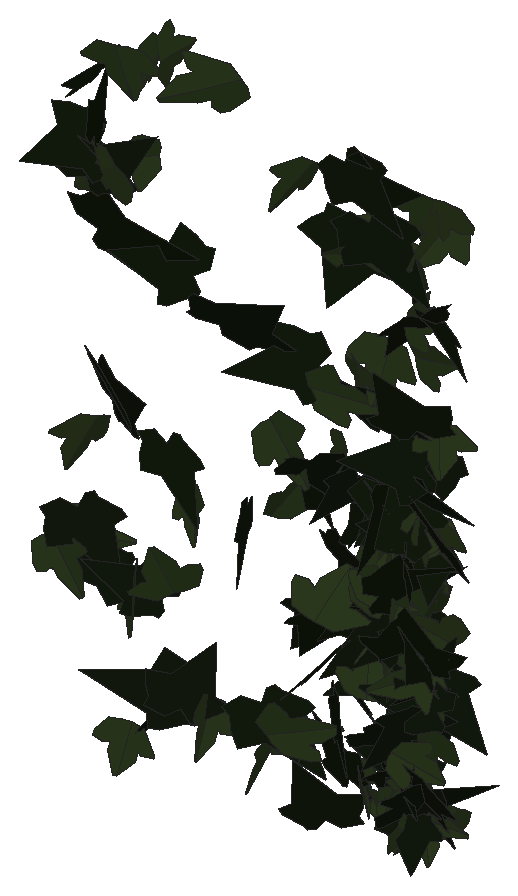
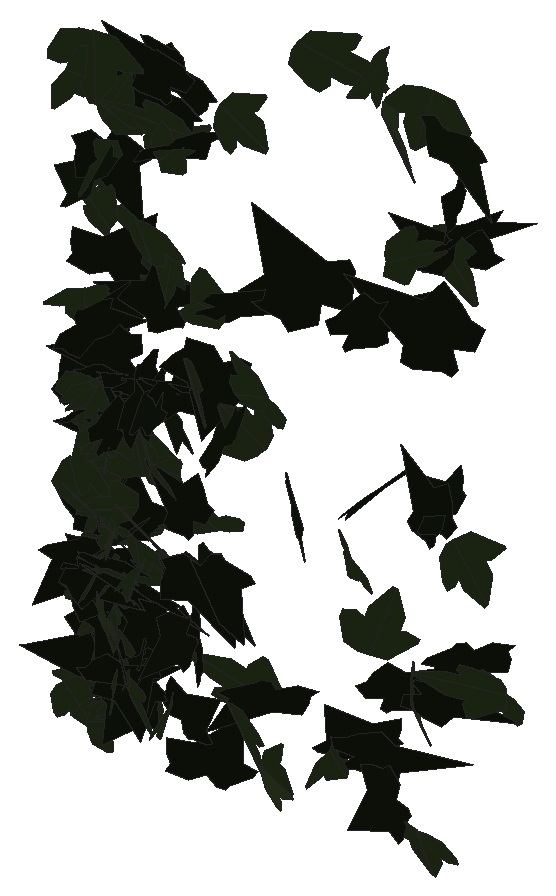
# SketchUp Ruby script. Lengths in inches.
U = 1.inch
M = Sketchup.active_model
def pt(a) = Geom::Point3d.new(a.map { |v| v * U })
def face(e, loops, mat)
  f = e.add_face(loops[0].map { |a| pt(a) })
  loops[1..].each { |l| e.add_face(l.map { |a| pt(a) }).erase! }
  f.material = f.back_material = mat if mat
  f
end
# faces: each face lists its corners as indices into pts; further lists are holes
def faces(e, pts, list, mat = nil) = list.each { |f| face(e, (f[0].is_a?(Array) ? f : [f]).map { |l| l.map { |i| pts[i] } }, mat) }
# xy, xz, yz: faces in a plane at the given z, y or x. An outline is a flat list of corners, or four numbers for a rectangle; further outlines are holes
def ring(l) = l.size == 4 ? [[l[0], l[1]], [l[2], l[1]], [l[2], l[3]], [l[0], l[3]]] : l.each_slice(2).to_a
def flat(e, list, mat, &to3) = list.each { |f| face(e, (f[0].is_a?(Array) ? f : [f]).map { |l| ring(l).map { |u, v| to3.(u, v) } }, mat) }
def xy(e, z, list, mat = nil) = flat(e, list, mat) { |x, y| [x, y, z] }
def xz(e, y, list, mat = nil) = flat(e, list, mat) { |x, z| [x, y, z] }
def yz(e, x, list, mat = nil) = flat(e, list, mat) { |y, z| [x, y, z] }
def lines(e, pts, list) = list.each { |a, b| e.add_line(pt(pts[a]), pt(pts[b])) }
# prism: a flat outline (further loops are holes) pulled along v
def prism(e, loops, v, mat = nil)
  f = face(e, loops, mat); d = Geom::Vector3d.new(v.map { |x| x * U })
  f.pushpull(f.normal.samedirection?(d) ? d.length : -d.length)
end
def box(e, o, s, mat = nil) = prism(e, [[o, [o[0] + s[0], o[1], o[2]], [o[0] + s[0], o[1] + s[1], o[2]], [o[0], o[1] + s[1], o[2]]]], [0, 0, s[2]], mat)
def at(x, y, z, deg = 0) = Geom::Transformation.translation(pt([x, y, z])) * Geom::Transformation.rotation(ORIGIN, Z_AXIS, deg.degrees)
def axes(o, x, y, z) = Geom::Transformation.new([*x, 0, *y, 0, *z, 0, *pt(o).to_a, 1])
def part(name) = M.definitions.add(name)
# library, detail: a bought-in or finely detailed component or shape, given as its bounding box
def library(name, o, s) = part(name).tap { |d| box(d.entities, o, s) }
def detail(e, o, s) = box(e.add_group.entities, o, s)
def put(e, d, t, mat = nil) = e.add_instance(d, t).tap { |i| i.material = mat if mat }
def group(e, t, mat = nil) = e.add_group.tap { |g| g.transformation = t; g.material = mat if mat }.entities
root = M.entities
M.materials.add("1026 AP 7946 SUNNY SIDE UP").color = [254, 231, 186]
M.materials.add("efeu1").color = [18, 25, 13]
M.materials.add("efeu2").color = [43, 57, 29]
c1 = part("ivyleaf_9")
p = [[1.54,2.16,1.25],[1.36,2.04,1.19],[-0.21,0.99,0.68],[-0.71,1.11,0.82],[-0.85,0.86,0.67],[-0.8,0.17,0.21],
  [-0.9,-0.01,0.1],[-0.67,-0.16,-0.02],[-0.08,-0.08,-0.05],[-0.03,-0.6,-0.4],[0.65,-0.88,-0.66],[0.83,-0.6,-0.49],
  [1.29,-0.42,-0.43],[1.8125,-0.07,-0.26],[1.21,0.44,0.15]]
faces(c1.entities,p,[[0,1,2,3,4,5,6,7,8,9,10,11,12,13,14]],"efeu1")
c2 = part("ivyleaf_10")
p = [[0,0.5,-0.03],[-0.0625,2.02,-0.43],[-0.19,2.01,-0.46],[-0.54,1.05,-0.29],[-0.52,0.625,-0.18],[-0.83,0.76,-0.28],
  [-1.16,0.64,-0.33],[-1.15,0.33,-0.24],[-0.77,-0.39,0.02],[-0.3,-0.51,0.16],[0.04,-0.48,0.23],[-0.02,2.01,-0.4375],
  [-0.06,2.01,-0.43],[0.04,-0.49,0.23],[0.67,-0.49,0.14],[1.38,0.36,-0.2],[1.375,0.51,-0.24],[0.81,0.65,-0.19],
  [0.62,0.59,-0.15],[0.6,1.09,-0.28],[0.5,1.23,-0.31]]
faces(c2.entities,p,[[0,1,2,3,4,5,6,7,8,9,10],[11,12,0,13,14,15,16,17,18,19,20]],"efeu2")
put(root,c1,axes([136.73,210.17,270.59],[-0.26614,0.28728,-0.15175],[0.0914,-0.13835,-0.34379],[-0.50054,-0.17801,0.01791]),"1026 AP 7946 SUNNY SIDE UP")
put(root,c1,axes([134.75,210.21,275.29],[0.64313,0.07781,-0.06027],[0.07787,0.05342,0.42695],[0.13227,-0.40977,0.04169]),"1026 AP 7946 SUNNY SIDE UP")
put(root,c1,axes([138.13,210.27,268.39],[-0.27927,-0.11413,-0.14956],[0.23344,0.03006,-0.21224],[0.17132,-0.227,0.0454]),"1026 AP 7946 SUNNY SIDE UP")
put(root,c1,axes([137.875,209.9,272.13],[0.11299,0.0966,0.37841],[0.47621,0.2101,-0.11691],[-0.35901,0.3091,-0.03598]),"1026 AP 7946 SUNNY SIDE UP")
put(root,c1,axes([138.1,210.46,271.06],[-0.02512,-0.18644,0.31261],[-0.05138,-0.30277,-0.19451],[0.55907,-0.03621,-0.00383]),"1026 AP 7946 SUNNY SIDE UP")
put(root,c2,axes([134.65,210.36,279.11],[-0.23805,-0.09443,0.34964],[-0.35505,-0.25829,-0.17903],[0.42625,-0.26788,0.04614]),"1026 AP 7946 SUNNY SIDE UP")
put(root,c2,axes([138.25,210.43,270.72],[0.13107,0.05274,-0.3635],[-0.35701,-0.27206,-0.09866],[-0.43333,0.2401,-0.02867]),"1026 AP 7946 SUNNY SIDE UP")
put(root,c1,axes([132.18,210.5,277.25],[-0.2853,-0.16132,0.29209],[-0.28268,-0.22252,-0.24944],[0.42951,-0.2536,0.02985]),"1026 AP 7946 SUNNY SIDE UP")
put(root,c1,axes([133.65,210.33,272.86],[0.10695,-0.35729,-0.04746],[-0.02162,0.04221,-0.3744],[0.56564,0.06917,-0.00534]),"1026 AP 7946 SUNNY SIDE UP")
put(root,c2,axes([135.89,210.13,272.75],[-0.05032,-0.28781,0.17373],[0.02448,0.16958,0.29931],[-0.52525,0.03548,-0.00269]),"1026 AP 7946 SUNNY SIDE UP")
put(root,c2,axes([133.69,210.36,270.61],[-0.30833,-0.26039,-0.16424],[-0.18219,-0.10995,0.33427],[-0.44287,0.22652,-0.02316]),"1026 AP 7946 SUNNY SIDE UP")
put(root,c2,axes([138.125,210.37,268.875],[-0.10338,-0.1906,0.18428],[-0.07209,-0.17431,-0.20847],[0.40582,-0.07952,0.00991]),"1026 AP 7946 SUNNY SIDE UP")
put(root,c1,axes([138.22,210.375,269.99],[-0.01066,0.16452,-0.33169],[-0.00555,-0.32297,-0.17134],[-0.56981,0.00007,0.00788]),"1026 AP 7946 SUNNY SIDE UP")
put(root,c1,axes([136.56,210.45,269.68],[-0.03088,-0.02035,-0.38486],[0.54423,-0.14274,-0.01158],[-0.22291,-0.34568,0.02506]),"1026 AP 7946 SUNNY SIDE UP")
put(root,c2,axes([138.13,210.07,269.46],[0.12399,0.16893,0.25185],[0.1136,0.23342,-0.18956],[-0.45195,0.10502,0.02144]),"1026 AP 7946 SUNNY SIDE UP")
put(root,c1,axes([134.97,210.46,272.2],[-0.19885,0.023,-0.35438],[0.47826,-0.16535,-0.12751],[-0.25566,-0.32722,0.03711]),"1026 AP 7946 SUNNY SIDE UP")
put(root,c1,axes([133.89,210.39,268.8],[-0.27735,0.03023,0.33699],[-0.51531,-0.03891,-0.17867],[0.03157,-0.36945,0.04419]),"1026 AP 7946 SUNNY SIDE UP")
put(root,c2,axes([135.83,210.19,269.01],[-0.25935,-0.06483,0.30417],[0.39299,0.1607,0.1809],[-0.26838,0.29795,-0.02905]),"1026 AP 7946 SUNNY SIDE UP")
put(root,c2,axes([137.25,210.25,271.875],[-0.00984,0.02412,0.31447],[0.46837,0.07065,0.00095],[-0.11066,0.29689,-0.02393]),"1026 AP 7946 SUNNY SIDE UP")
put(root,c1,axes([138.06,210.5625,273.98],[-0.18142,-0.07753,0.38218],[-0.43482,-0.24863,-0.14341],[0.40851,-0.29908,0.01708]),"1026 AP 7946 SUNNY SIDE UP")
put(root,c2,axes([131.58,210.34,270.52],[0.37526,-0.01701,0.23964],[0.36328,-0.02943,-0.24647],[0.05143,0.33203,-0.00761]),"1026 AP 7946 SUNNY SIDE UP")
put(root,c1,axes([136.43,210.13,273.68],[0.30385,0.27277,-0.0482],[-0.02167,-0.04939,-0.34421],[-0.43505,0.19297,-0.01652]),"1026 AP 7946 SUNNY SIDE UP")
put(root,c2,axes([132.83,210.28,278.96],[-0.52336,-0.04407,-0.04314],[0.07175,-0.0292,-0.34421],[0.06275,-0.33416,0.03377]),"1026 AP 7946 SUNNY SIDE UP")
put(root,c2,axes([132.86,210.37,267.92],[0.47079,-0.06296,0.02228],[0.02472,-0.03166,-0.31409],[0.10191,0.29854,-0.02676]),"1026 AP 7946 SUNNY SIDE UP")
put(root,c1,axes([137.97,210.37,270.9],[0.51186,0.03665,0.18094],[-0.28073,0.03454,0.33405],[0.02463,-0.36817,0.04716]),"1026 AP 7946 SUNNY SIDE UP")
put(root,c2,axes([137.99,210.44,272.24],[0.15379,0.23935,-0.21078],[-0.09836,-0.19665,-0.26719],[-0.48667,0.11538,-0.01261]),"1026 AP 7946 SUNNY SIDE UP")
put(root,c1,axes([138.04,210.22,269.12],[0.63379,-0.06727,-0.16095],[-0.24931,-0.00577,-0.41991],[0.09533,0.43212,-0.02808]),"1026 AP 7946 SUNNY SIDE UP")
put(root,c2,axes([135.49,210.44,273.6875],[0.33715,-0.01288,0.33394],[0.49072,-0.09821,-0.21722],[0.13969,0.3761,-0.04293]),"1026 AP 7946 SUNNY SIDE UP")
put(root,c1,axes([138.08,210.4,274.6875],[0.2781,0.01571,0.27956],[-0.42679,0.02574,0.18092],[-0.0205,-0.32282,0.02613]),"1026 AP 7946 SUNNY SIDE UP")
put(root,c1,axes([137.61,210.56,268.89],[0.09588,-0.22587,0.23585],[0.08395,-0.224,-0.24228],[0.50014,0.0809,-0.00455]),"1026 AP 7946 SUNNY SIDE UP")
put(root,c2,axes([137.99,210.2,268.24],[-0.06269,-0.1766,-0.22164],[0.12216,0.20059,-0.18415],[0.41901,-0.08491,0.02053]),"1026 AP 7946 SUNNY SIDE UP")
put(root,c1,axes([138.45,210.36,270.23],[-0.25328,0.0694,0.2497],[-0.37256,0.05528,-0.17849],[-0.13376,-0.28539,0.02432]),"1026 AP 7946 SUNNY SIDE UP")
put(root,c1,axes([134.01,210.2,268.83],[-0.29691,-0.04659,0.28487],[0.39529,0.1203,0.19824],[-0.1963,0.31272,-0.03168]),"1026 AP 7946 SUNNY SIDE UP")
put(root,c1,axes([136.92,210.49,273.4],[-0.04346,0.10021,-0.27693],[0.0868,-0.26374,-0.10845],[-0.44353,-0.06143,0.00592]),"1026 AP 7946 SUNNY SIDE UP")
put(root,c2,axes([134.3,210.5,268.74],[0.06042,0.28703,-0.22609],[-0.06918,-0.21699,-0.29935],[-0.56548,0.05721,0.01247]),"1026 AP 7946 SUNNY SIDE UP")
put(root,c1,axes([138.32,210.34,268.61],[0.12464,-0.0563,0.25825],[-0.29095,0.16998,0.10047],[-0.28099,-0.20098,0.01052]),"1026 AP 7946 SUNNY SIDE UP")
put(root,c1,axes([138.06,210.24,272.6],[0.17787,-0.10591,-0.28495],[-0.35878,0.15661,-0.15734],[0.29554,0.25386,-0.01952]),"1026 AP 7946 SUNNY SIDE UP")
put(root,c2,axes([137.28,210.29,270.23],[0.35223,0.16172,-0.04466],[0.03139,0.04762,0.28359],[0.26177,-0.22332,0.02608]),"1026 AP 7946 SUNNY SIDE UP")
put(root,c1,axes([138,210.09,268.62],[0.11303,0.31226,-0.27155],[0.04457,0.26498,0.33068],[0.6428,-0.07328,0.02482]),"1026 AP 7946 SUNNY SIDE UP")
put(root,c2,axes([138.37,210.35,269.82],[-0.48773,0.03857,0.12281],[-0.19078,-0.0154,-0.32078],[-0.04783,-0.33187,0.02718]),"1026 AP 7946 SUNNY SIDE UP")
put(root,c1,axes([137.25,210.45,277.66],[-0.13024,-0.14572,-0.36707],[0.52719,0.15015,-0.14301],[0.29498,-0.33269,0.09352]),"1026 AP 7946 SUNNY SIDE UP")
put(root,c1,axes([132.47,210.26,278.6],[-0.17953,0.34768,0.01294],[-0.02468,0.00598,-0.37672],[-0.54639,-0.11451,0.01276]),"1026 AP 7946 SUNNY SIDE UP")
put(root,c1,axes([136.08,210.62,274.91],[-0.38108,-0.0838,0.26753],[-0.34164,-0.1519,-0.2598],[0.26076,-0.32148,0.05059]),"1026 AP 7946 SUNNY SIDE UP")
put(root,c2,axes([136.52,210.22,271.27],[0.46457,0.1013,-0.15908],[0.14876,0.1683,0.3001],[0.25027,-0.28808,0.11692]),"1026 AP 7946 SUNNY SIDE UP")
put(root,c1,axes([135.37,210.35,269.24],[0.03333,-0.25357,-0.28363],[0.11211,0.27202,-0.25217],[0.57607,-0.03827,0.06549]),"1026 AP 7946 SUNNY SIDE UP")
put(root,c2,axes([132.58,210.35,276.98],[-0.41771,0.07158,0.26406],[-0.40832,0.0069,-0.27964],[-0.08871,-0.3688,0.04378]),"1026 AP 7946 SUNNY SIDE UP")
put(root,c1,axes([138.15,210.37,276.5],[-0.03699,0.31016,-0.14915],[0.0141,-0.14628,-0.32129],[-0.5392,-0.0251,0.00183]),"1026 AP 7946 SUNNY SIDE UP")
put(root,c1,axes([137.39,210.72,273.2],[-0.04348,-0.01088,-0.46251],[0.46618,-0.33821,-0.01234],[-0.53026,-0.29645,0.02707]),"1026 AP 7946 SUNNY SIDE UP")
put(root,c2,axes([137.78,210.33,268.42],[0.0358,0.01827,0.38531],[0.53357,0.1572,-0.02828],[-0.24861,0.34003,-0.00521]),"1026 AP 7946 SUNNY SIDE UP")
put(root,c1,axes([137.34,210.23,269.54],[0.28308,0.18338,0.10229],[0.13226,0.05467,-0.26359],[-0.29919,0.19767,-0.01975]),"1026 AP 7946 SUNNY SIDE UP")
put(root,c2,axes([137.6,210.3125,271.8],[0.4458,0.18264,-0.07887],[0.07595,0.06772,0.34646],[0.30264,-0.28603,0.02922]),"1026 AP 7946 SUNNY SIDE UP")
put(root,c2,axes([137.34,210.44,268.4],[-0.28245,0.15267,-0.1004],[0.09622,-0.07932,-0.24252],[-0.26884,-0.18879,0.01868]),"1026 AP 7946 SUNNY SIDE UP")
put(root,c2,axes([136.43,210.39,274.68],[-0.08928,0.00465,0.35232],[0.51863,0.09238,0.05566],[-0.14215,0.33411,-0.01819]),"1026 AP 7946 SUNNY SIDE UP")
put(root,c1,axes([136.38,210.48,267.73],[0.26833,0.08542,0.26178],[-0.4152,0.0048,0.1814],[0.06847,-0.30565,0.07408]),"1026 AP 7946 SUNNY SIDE UP")
put(root,c2,axes([138.46,210.6,271.29],[-0.21494,-0.15184,-0.27938],[-0.34525,-0.16119,0.2067],[-0.34422,0.25648,-0.03287]),"1026 AP 7946 SUNNY SIDE UP")
put(root,c2,axes([132.05,210.55,272.5625],[-0.13776,-0.34154,0.11707],[-0.02345,-0.11541,-0.36365],[0.56647,-0.08784,0.01342]),"1026 AP 7946 SUNNY SIDE UP")
put(root,c2,axes([136.91,210.68,276.97],[-0.07115,-0.06947,-0.31803],[-0.22034,-0.27477,0.08336],[-0.44544,0.14701,0.00957]),"1026 AP 7946 SUNNY SIDE UP")
put(root,c1,axes([132.23,210.33,276.79],[-0.15861,0.02976,0.32855],[0.50332,0.01482,0.10301],[-0.00821,0.334,-0.03187]),"1026 AP 7946 SUNNY SIDE UP")
put(root,c2,axes([137.39,210.57,275.6],[0.56896,-0.11957,0.04142],[0.04608,-0.04123,-0.39163],[0.19328,0.3618,-0.02857]),"1026 AP 7946 SUNNY SIDE UP")
put(root,c1,axes([137.65,210.64,273.2],[-0.40454,-0.12657,0.01914],[-0.00818,-0.03295,-0.29424],[0.20115,-0.25588,0.02654]),"1026 AP 7946 SUNNY SIDE UP")
put(root,c1,axes([138.07,210.51,273.02],[-0.44402,-0.18993,-0.17658],[-0.25408,-0.06345,0.34851],[-0.31041,0.32361,-0.03268]),"1026 AP 7946 SUNNY SIDE UP")
put(root,c1,axes([137.58,210.4375,269.24],[0.29218,-0.12814,-0.15735],[-0.2256,0.05762,-0.23037],[0.21642,0.23306,-0.0277]),"1026 AP 7946 SUNNY SIDE UP")
put(root,c2,axes([138.23,210.63,271.92],[-0.07504,-0.35159,0.14809],[-0.00667,-0.14639,-0.36608],[0.59842,-0.04572,0.01449]),"1026 AP 7946 SUNNY SIDE UP")
put(root,c1,axes([137.84,210.36,269.44],[0.29876,0.18475,0.00136],[0.02017,-0.0128,-0.27245],[-0.28981,0.18957,-0.01755]),"1026 AP 7946 SUNNY SIDE UP")
put(root,c1,axes([136.75,210.76,277.17],[-0.28079,-0.33585,0.08636],[-0.02977,-0.08685,-0.39162],[0.54422,-0.17803,0.02314]),"1026 AP 7946 SUNNY SIDE UP")
put(root,c1,axes([135.87,210.77,272.97],[0.29081,-0.17782,-0.2867],[0.35119,-0.16606,0.26219],[-0.38073,-0.289,0.02286]),"1026 AP 7946 SUNNY SIDE UP")
put(root,c2,axes([138.18,210.5,268.17],[0.11528,0.23643,-0.02662],[-0.00166,-0.02812,-0.25506],[-0.3742,0.07296,-0.00707]),"1026 AP 7946 SUNNY SIDE UP")
put(root,c1,axes([137.75,210.74,270.8],[-0.12014,-0.21094,0.19055],[-0.0125,-0.19121,-0.22768],[0.4422,-0.06271,0.04533]),"1026 AP 7946 SUNNY SIDE UP")
put(root,c2,axes([138.3125,210.45,270.25],[0.14915,-0.06816,-0.26612],[-0.36169,0.11778,-0.11852],[0.21251,0.2483,-0.01494]),"1026 AP 7946 SUNNY SIDE UP")
put(root,c2,axes([137.11,210.69,272.19],[0.36911,-0.14025,0.27182],[0.30546,-0.18463,-0.2794],[0.35847,0.30175,-0.04181]),"1026 AP 7946 SUNNY SIDE UP")
put(root,c1,axes([138.4,210.6,272.73],[0.29423,-0.29874,0.18965],[-0.12962,0.16734,0.36372],[-0.53777,-0.20378,0.0161]),"1026 AP 7946 SUNNY SIDE UP")
put(root,c2,axes([137.07,210.47,275.1875],[-0.41398,0.17699,0.04124],[-0.07851,-0.00466,-0.32523],[-0.27395,-0.26611,0.03087]),"1026 AP 7946 SUNNY SIDE UP")
put(root,c1,axes([138.1,210.32,269.375],[-0.07557,0.00756,-0.34682],[-0.47051,0.15511,0.04849],[0.243,0.30268,-0.01396]),"1026 AP 7946 SUNNY SIDE UP")
put(root,c2,axes([137.91,210.7,269.83],[0.03658,-0.20463,0.20217],[0.10227,-0.18899,-0.21082],[0.43523,0.06161,0.03255]),"1026 AP 7946 SUNNY SIDE UP")
put(root,c2,axes([138,210.48,277.14],[-0.42318,0.17665,-0.11522],[-0.12491,0.084,0.33112],[0.30502,0.27948,-0.02426]),"1026 AP 7946 SUNNY SIDE UP")
put(root,c1,axes([138.15,210.6875,272.67],[-0.12286,-0.27832,0.0111],[0.00789,-0.01424,-0.29775],[0.43798,-0.07781,0.00848]),"1026 AP 7946 SUNNY SIDE UP")
put(root,c2,axes([132.65,210.76,270.16],[0.23681,-0.17536,0.32947],[0.3335,-0.24071,-0.23953],[0.46827,0.26012,0.00397]),"1026 AP 7946 SUNNY SIDE UP")
put(root,c1,axes([137.17,210.33,272.86],[-0.23097,0.0674,-0.26752],[-0.33571,0.15062,0.16533],[0.2564,0.25792,-0.02451]),"1026 AP 7946 SUNNY SIDE UP")
put(root,c1,axes([136.9,210.5625,274.6],[0.29094,-0.06199,0.22944],[0.3002,-0.12068,-0.1984],[0.20594,0.2635,-0.03494]),"1026 AP 7946 SUNNY SIDE UP")
put(root,c2,axes([137.95,210.79,268.0625],[0.01537,-0.09049,0.32955],[0.09327,-0.31494,-0.09534],[0.51514,0.05972,0.00743]),"1026 AP 7946 SUNNY SIDE UP")
put(root,c2,axes([135.78,210.72,277.93],[-0.05215,-0.27539,0.21292],[-0.02696,-0.20763,-0.2869],[0.54222,-0.03681,0.00621]),"1026 AP 7946 SUNNY SIDE UP")
put(root,c2,axes([133.76,210.68,271.9],[0.3071,-0.12001,0.21594],[0.26128,-0.13007,-0.23622],[0.2769,0.25583,-0.0166]),"1026 AP 7946 SUNNY SIDE UP")
put(root,c1,axes([138.16,210.45,270.32],[0.14353,0.25165,-0.06108],[-0.02223,-0.05944,-0.27603],[-0.40644,0.09212,-0.00647]),"1026 AP 7946 SUNNY SIDE UP")
put(root,c1,axes([132.16,210.78,273.25],[0.11308,-0.2263,0.26656],[0.11042,-0.25044,-0.246],[0.53066,0.10034,-0.00561]),"1026 AP 7946 SUNNY SIDE UP")
put(root,c1,axes([131.88,210.53,271.125],[-0.01622,-0.27492,-0.25137],[0.01182,0.24233,-0.282],[0.57624,-0.01271,-0.00129]),"1026 AP 7946 SUNNY SIDE UP")
put(root,c2,axes([133.62,210.29,279.22],[0.0346,-0.05695,-0.36877],[0.10546,0.35274,-0.05155],[0.55959,-0.06296,0.03251]),"1026 AP 7946 SUNNY SIDE UP")
put(root,c1,axes([133.16,210.71,270.11],[-0.05961,0.03673,0.34222],[-0.49032,-0.12359,-0.02332],[0.18815,-0.31044,0.04764]),"1026 AP 7946 SUNNY SIDE UP")
put(root,c1,axes([132.3,210.36,277.5],[-0.04261,-0.07348,0.33653],[0.17172,0.30831,0.08248],[-0.49837,0.11252,-0.00035]),"1026 AP 7946 SUNNY SIDE UP")
put(root,c1,axes([132.55,210.69,270.32],[-0.12236,-0.10405,-0.28652],[-0.26869,-0.2187,0.13255],[-0.38081,0.18774,-0.00146]),"1026 AP 7946 SUNNY SIDE UP")
put(root,c1,axes([132.33,210.76,272.98],[-0.01399,-0.02126,0.38076],[0.19042,-0.34966,-0.01975],[0.55029,0.12045,0.01652]),"1026 AP 7946 SUNNY SIDE UP")
put(root,c2,axes([135.11,210.76,268.28],[0.15126,-0.23356,0.22129],[0.10025,-0.20707,-0.26096],[0.49022,0.11441,-0.01491]),"1026 AP 7946 SUNNY SIDE UP")
put(root,c1,axes([137.45,210.66,271.16],[-0.60423,0.14588,-0.1043],[0.12757,-0.07266,-0.42205],[-0.24921,-0.3909,0.03684]),"1026 AP 7946 SUNNY SIDE UP")
put(root,c1,axes([133.67,210.81,275.46],[-0.10197,-0.00874,0.39409],[-0.48887,-0.22504,-0.06091],[0.35084,-0.31612,0.02967]),"1026 AP 7946 SUNNY SIDE UP")
put(root,c1,axes([132.18,210.68,275.72],[0.2045,-0.0656,0.4257],[0.50475,-0.2625,-0.14841],[0.42285,0.34506,-0.02872]),"1026 AP 7946 SUNNY SIDE UP")
put(root,c1,axes([137.67,210.6,273.55],[0.33403,-0.08508,0.1851],[0.25562,-0.07824,-0.236],[0.18112,0.26733,-0.0083]),"1026 AP 7946 SUNNY SIDE UP")
put(root,c2,axes([137.97,210.68,275.64],[-0.22788,0.07635,0.30345],[0.45192,-0.07136,0.16456],[0.15514,0.32003,-0.03363]),"1026 AP 7946 SUNNY SIDE UP")
put(root,c1,axes([137.92,210.73,270.24],[-0.43063,-0.05853,-0.06874],[0.1144,-0.02591,-0.28578],[0.07927,-0.2806,0.039]),"1026 AP 7946 SUNNY SIDE UP")
put(root,c2,axes([137.89,210.57,270.1],[-0.19892,-0.10465,-0.21233],[0.33933,0.02895,-0.15187],[0.12789,-0.23958,0.07271]),"1026 AP 7946 SUNNY SIDE UP")
put(root,c2,axes([138.13,210.7,273.02],[0.27167,0.19318,-0.13302],[-0.10541,-0.11403,-0.26658],[-0.35082,0.18386,-0.0229]),"1026 AP 7946 SUNNY SIDE UP")
put(root,c1,axes([137.4375,210.54,269.12],[0.23388,-0.02503,-0.22362],[-0.34013,0.01899,-0.15494],[0.04694,0.26233,-0.00856]),"1026 AP 7946 SUNNY SIDE UP")
put(root,c1,axes([137.93,210.75,270.49],[-0.35508,-0.12648,-0.05556],[0.09955,-0.00512,-0.26427],[0.19143,-0.23195,0.03437]),"1026 AP 7946 SUNNY SIDE UP")
put(root,c1,axes([136.62,210.7,278.3],[-0.06251,-0.09717,-0.34855],[0.52079,0.10344,-0.07021],[0.18501,-0.324,0.07986]),"1026 AP 7946 SUNNY SIDE UP")
put(root,c2,axes([136.94,210.61,277.28],[0.06683,-0.03585,-0.33407],[0.51219,-0.00984,0.04507],[-0.02276,-0.32671,0.03337]),"1026 AP 7946 SUNNY SIDE UP")
put(root,c2,axes([136.59,210.55,273.7],[0.17826,-0.23479,-0.19294],[-0.1228,0.16878,-0.2676],[0.45466,0.13764,0.00337]),"1026 AP 7946 SUNNY SIDE UP")
put(root,c2,axes([137.48,210.49,268.34],[0.09731,0.07064,0.24985],[0.21347,0.20077,-0.09492],[-0.33423,0.1488,0.01211]),"1026 AP 7946 SUNNY SIDE UP")
put(root,c1,axes([136.87,210.72,278.03],[0.0513,-0.00636,0.32549],[0.34867,-0.22589,-0.02959],[0.35411,0.22334,-0.01802]),"1026 AP 7946 SUNNY SIDE UP")
put(root,c1,axes([137.24,210.7,270.26],[-0.40373,0.04838,0.03375],[-0.05535,-0.01181,-0.2686],[-0.07303,-0.25854,0.01702]),"1026 AP 7946 SUNNY SIDE UP")
put(root,c2,axes([138.1,210.68,272.96],[0.10453,0.27439,-0.07754],[-0.01393,-0.07686,-0.29114],[-0.44782,0.06644,-0.00904]),"1026 AP 7946 SUNNY SIDE UP")
put(root,c2,axes([137.32,210.73,270.92],[0.39962,-0.07196,0.08405],[0.11071,-0.0506,-0.27086],[0.13103,0.26221,-0.0275]),"1026 AP 7946 SUNNY SIDE UP")
put(root,c2,axes([137.91,210.58,269.24],[0.29501,-0.12811,-0.17486],[-0.15163,0.14944,-0.22611],[0.297,0.20355,0.05825]),"1026 AP 7946 SUNNY SIDE UP")
put(root,c2,axes([136.9,210.69,268.57],[-0.08496,0.28251,-0.09695],[0.0206,-0.09493,-0.29683],[-0.46857,-0.0554,0.00453]),"1026 AP 7946 SUNNY SIDE UP")
put(root,c2,axes([137.9375,210.72,269.86],[0.07932,-0.25559,0.02896],[0.0059,-0.02939,-0.26855],[0.40453,0.05055,-0.00176]),"1026 AP 7946 SUNNY SIDE UP")
put(root,c2,axes([137.71,210.6,268.82],[0.02969,-0.25103,-0.12555],[0.0899,0.12165,-0.25124],[0.42848,-0.00813,0.06142]),"1026 AP 7946 SUNNY SIDE UP")
put(root,c1,axes([136.69,210.6,268.48],[0.09698,-0.06919,0.276],[-0.21527,0.23136,0.09524],[-0.37878,-0.1492,0.01653]),"1026 AP 7946 SUNNY SIDE UP")
put(root,c2,axes([137.93,210.67,272.46],[-0.38206,-0.0209,-0.13597],[0.2099,-0.03275,-0.24823],[0.00405,-0.27451,0.03833]),"1026 AP 7946 SUNNY SIDE UP")
put(root,c1,axes([138.16,210.95,274.04],[0.00275,-0.12571,-0.32902],[0.11359,-0.31136,0.12513],[-0.52653,-0.06783,0.02527]),"1026 AP 7946 SUNNY SIDE UP")
put(root,c2,axes([131.59,210.6,270.68],[0.03832,-0.05803,-0.35269],[0.5398,0.05339,0.01618],[0.07852,-0.33871,0.06089]),"1026 AP 7946 SUNNY SIDE UP")
put(root,c1,axes([133.3125,210.39,268.34],[0.12751,0.18232,0.29102],[0.18399,0.25598,-0.20406],[-0.49415,0.14236,-0.00089]),"1026 AP 7946 SUNNY SIDE UP")
put(root,c2,axes([137.78,210.49,271.24],[-0.02813,-0.01088,0.28642],[0.09509,0.27185,0.01656],[-0.42715,0.06124,-0.01518]),"1026 AP 7946 SUNNY SIDE UP")
put(root,c2,axes([137.89,210.68,270.91],[-0.22698,0.21919,-0.05018],[0.02875,-0.04772,-0.27043],[-0.35232,-0.14511,0.01026]),"1026 AP 7946 SUNNY SIDE UP")
put(root,c1,axes([138.25,210.79,270.25],[-0.16494,0.11927,-0.21148],[0.00944,-0.22368,-0.1379],[-0.37411,-0.05823,0.08976]),"1026 AP 7946 SUNNY SIDE UP")
put(root,c1,axes([138.09,210.61,270.48],[-0.06414,-0.20871,-0.33973],[0.1244,0.31905,-0.21702],[0.59932,-0.08856,0.00869]),"1026 AP 7946 SUNNY SIDE UP")
put(root,c2,axes([138.29,210.91,277.8],[0.13271,0.22612,-0.32987],[-0.22091,-0.28974,-0.24963],[-0.57719,0.16288,0.0197]),"1026 AP 7946 SUNNY SIDE UP")
put(root,c1,axes([136.35,210.86,271.74],[0.08373,-0.0757,0.3132],[0.23371,-0.26586,-0.09644],[0.43441,0.15762,-0.00848]),"1026 AP 7946 SUNNY SIDE UP")
put(root,c1,axes([138.28,210.79,271.29],[-0.40064,0.05505,-0.1023],[0.1405,-0.05452,-0.26681],[-0.11085,-0.26809,0.03155]),"1026 AP 7946 SUNNY SIDE UP")
put(root,c2,axes([138.43,210.8,268.36],[-0.18061,-0.21018,0.12151],[-0.06895,-0.1116,-0.24702],[0.37359,-0.12221,0.01315]),"1026 AP 7946 SUNNY SIDE UP")
put(root,c2,axes([138.04,210.45,276.33],[-0.01913,0.08193,0.33741],[-0.12041,0.31804,-0.08315],[-0.5163,-0.07721,0.00689]),"1026 AP 7946 SUNNY SIDE UP")
put(root,c1,axes([137.69,210.99,272.55],[-0.08553,-0.03052,0.39146],[-0.38051,-0.29404,-0.06171],[0.4635,-0.24702,0.02158]),"1026 AP 7946 SUNNY SIDE UP")
put(root,c2,axes([138.15,210.71,278.15],[-0.57095,-0.07429,0.04535],[-0.06093,-0.03186,-0.38125],[0.12172,-0.36443,0.02185]),"1026 AP 7946 SUNNY SIDE UP")
put(root,c1,axes([136.3,210.7,270.91],[0.09091,0.27104,-0.19786],[-0.04841,-0.1913,-0.2865],[-0.52149,0.06501,-0.00789]),"1026 AP 7946 SUNNY SIDE UP")
put(root,c1,axes([137.54,210.63,268.76],[0.14602,0.21927,-0.08849],[-0.0828,-0.07203,-0.24494],[-0.36165,0.10502,0.02035]),"1026 AP 7946 SUNNY SIDE UP")
put(root,c1,axes([136.27,210.73,270.9375],[0.20083,0.15156,-0.2685],[-0.24102,-0.21218,-0.20507],[-0.40959,0.19917,-0.01098]),"1026 AP 7946 SUNNY SIDE UP")
put(root,c1,axes([137.97,210.91,276.28],[0.16927,-0.29437,0.16188],[0.10009,-0.14575,-0.32363],[0.51632,0.12476,0.00967]),"1026 AP 7946 SUNNY SIDE UP")
put(root,c1,axes([137.8,210.83,268.75],[-0.07265,0.02946,0.29003],[-0.44056,-0.04419,-0.04289],[0.06152,-0.28169,0.03535]),"1026 AP 7946 SUNNY SIDE UP")
put(root,c2,axes([135.67,210.72,268.91],[0.35976,-0.27291,-0.144],[-0.15613,0.09702,-0.36607],[0.45498,0.24908,-0.01176]),"1026 AP 7946 SUNNY SIDE UP")
put(root,c1,axes([137.16,210.875,272.88],[0.26436,-0.22186,0.00384],[0.02413,0.01786,0.2859],[-0.34811,-0.16725,0.02273]),"1026 AP 7946 SUNNY SIDE UP")
put(root,c2,axes([132.98,210.85,278.8],[0.31938,-0.32397,0.0456],[0.01037,-0.0502,-0.39362],[0.51443,0.20214,-0.02038]),"1026 AP 7946 SUNNY SIDE UP")
put(root,c1,axes([137.49,210.59,268.49],[0.26175,0.18534,0.0458],[0.03429,0.03872,-0.25623],[-0.29735,0.16762,0.01077]),"1026 AP 7946 SUNNY SIDE UP")
put(root,c2,axes([132.77,210.99,276.97],[0.02163,-0.01084,-0.34641],[-0.3073,-0.27412,-0.00074],[-0.43049,0.19514,-0.01688]),"1026 AP 7946 SUNNY SIDE UP")
put(root,c2,axes([138.23,210.74,272.99],[-0.43466,0.08713,0.0281],[-0.05319,-0.01865,-0.29732],[-0.13309,-0.2771,0.02706]),"1026 AP 7946 SUNNY SIDE UP")
put(root,c2,axes([137.35,210.76,270.54],[-0.01676,0.26343,-0.02095],[0.00602,-0.02169,-0.27171],[-0.41559,-0.01094,-0.00309]),"1026 AP 7946 SUNNY SIDE UP")
put(root,c2,axes([137.52,210.6875,268.65],[0.16406,-0.13616,-0.21021],[-0.20213,0.15753,-0.17575],[0.32734,0.16551,-0.00316]),"1026 AP 7946 SUNNY SIDE UP")
put(root,c2,axes([138.2,210.8,274.43],[0.27395,0.23844,-0.03012],[-0.00837,-0.03395,-0.304],[-0.37791,0.1736,-0.01511]),"1026 AP 7946 SUNNY SIDE UP")
put(root,c2,axes([138.1,210.77,270.17],[-0.12109,0.24777,-0.03308],[0.004,-0.03429,-0.26738],[-0.39312,-0.07666,0.00747]),"1026 AP 7946 SUNNY SIDE UP")
put(root,c1,axes([136.55,210.76,269.85],[0.42025,-0.13497,-0.08023],[-0.12611,0.01164,-0.30731],[0.20937,0.27792,-0.02407]),"1026 AP 7946 SUNNY SIDE UP")
